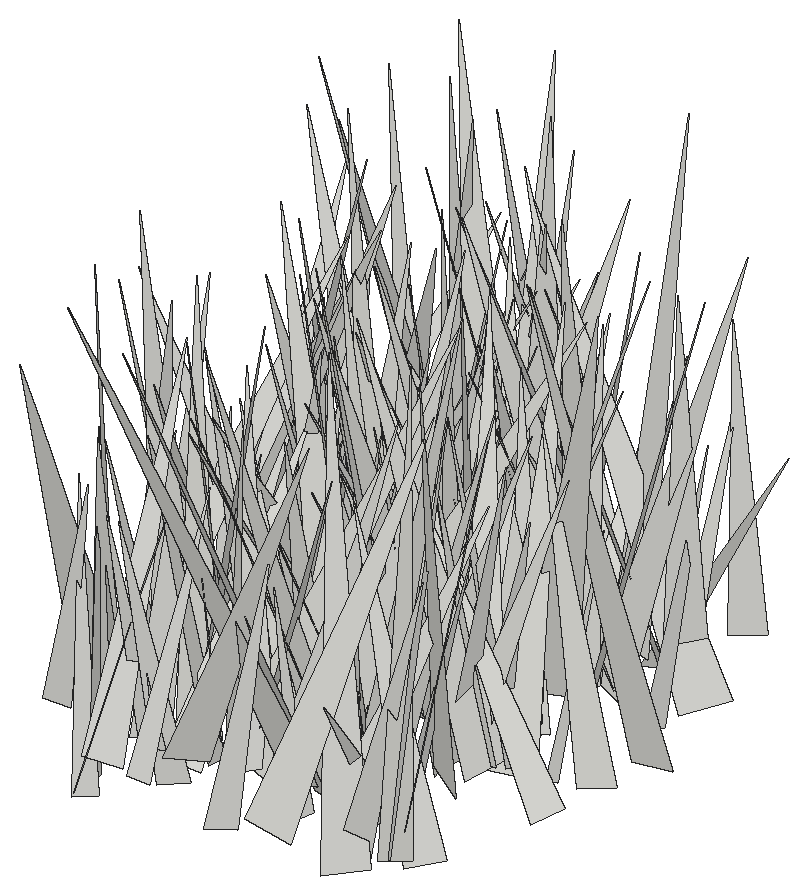
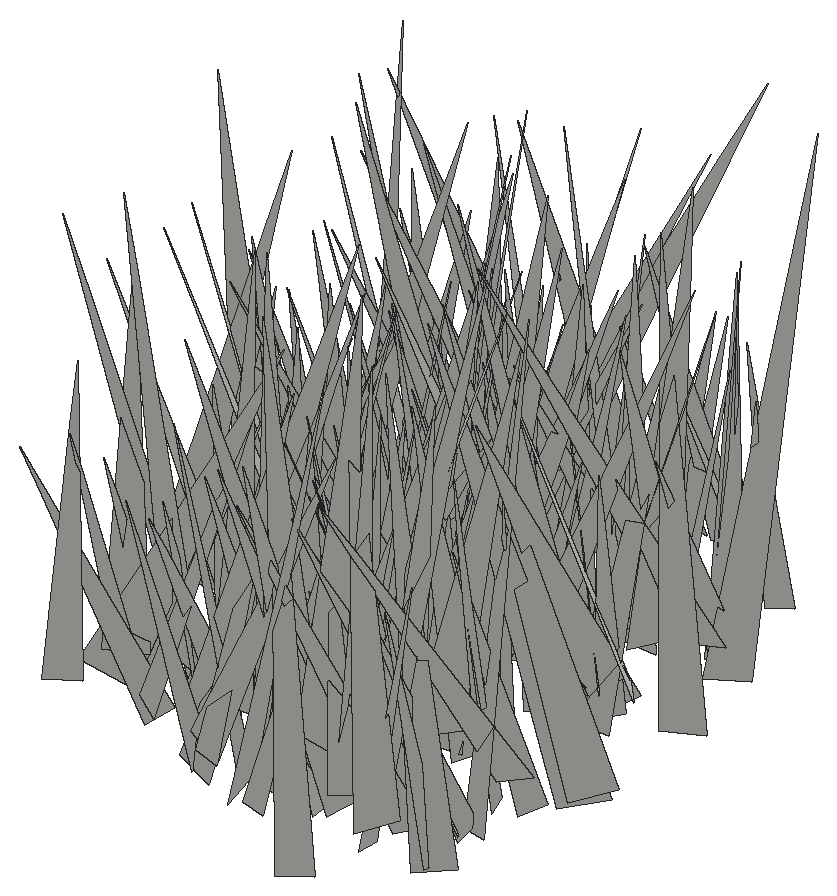
# SketchUp Ruby script. Lengths in inches.
U = 1.inch
M = Sketchup.active_model
def pt(a) = Geom::Point3d.new(a.map { |v| v * U })
def face(e, loops, mat)
  f = e.add_face(loops[0].map { |a| pt(a) })
  loops[1..].each { |l| e.add_face(l.map { |a| pt(a) }).erase! }
  f.material = f.back_material = mat if mat
  f
end
# faces: each face lists its corners as indices into pts; further lists are holes
def faces(e, pts, list, mat = nil) = list.each { |f| face(e, (f[0].is_a?(Array) ? f : [f]).map { |l| l.map { |i| pts[i] } }, mat) }
# xy, xz, yz: faces in a plane at the given z, y or x. An outline is a flat list of corners, or four numbers for a rectangle; further outlines are holes
def ring(l) = l.size == 4 ? [[l[0], l[1]], [l[2], l[1]], [l[2], l[3]], [l[0], l[3]]] : l.each_slice(2).to_a
def flat(e, list, mat, &to3) = list.each { |f| face(e, (f[0].is_a?(Array) ? f : [f]).map { |l| ring(l).map { |u, v| to3.(u, v) } }, mat) }
def xy(e, z, list, mat = nil) = flat(e, list, mat) { |x, y| [x, y, z] }
def xz(e, y, list, mat = nil) = flat(e, list, mat) { |x, z| [x, y, z] }
def yz(e, x, list, mat = nil) = flat(e, list, mat) { |y, z| [x, y, z] }
def lines(e, pts, list) = list.each { |a, b| e.add_line(pt(pts[a]), pt(pts[b])) }
# prism: a flat outline (further loops are holes) pulled along v
def prism(e, loops, v, mat = nil)
  f = face(e, loops, mat); d = Geom::Vector3d.new(v.map { |x| x * U })
  f.pushpull(f.normal.samedirection?(d) ? d.length : -d.length)
end
def box(e, o, s, mat = nil) = prism(e, [[o, [o[0] + s[0], o[1], o[2]], [o[0] + s[0], o[1] + s[1], o[2]], [o[0], o[1] + s[1], o[2]]]], [0, 0, s[2]], mat)
def at(x, y, z, deg = 0) = Geom::Transformation.translation(pt([x, y, z])) * Geom::Transformation.rotation(ORIGIN, Z_AXIS, deg.degrees)
def axes(o, x, y, z) = Geom::Transformation.new([*x, 0, *y, 0, *z, 0, *pt(o).to_a, 1])
def part(name) = M.definitions.add(name)
# library, detail: a bought-in or finely detailed component or shape, given as its bounding box
def library(name, o, s) = part(name).tap { |d| box(d.entities, o, s) }
def detail(e, o, s) = box(e.add_group.entities, o, s)
def put(e, d, t, mat = nil) = e.add_instance(d, t).tap { |i| i.material = mat if mat }
def group(e, t, mat = nil) = e.add_group.tap { |g| g.transformation = t; g.material = mat if mat }.entities
root = M.entities
c1 = part("fur_instance\#9")
p = [[0.8125,0,1.79],[0.67,-0.02,1.48],[0,-0.11,0],[0,0.11,0]]
faces(c1.entities,p,[[0,1,2,3]])
put(root,c1,axes([100.01,75.59,-28.22],[-2.89622,3.26829,0.45856],[3.08153,2.89643,-1.18106],[1.18158,0.4572,4.20415]))
put(root,c1,axes([98.46,79.53,-28.22],[1.17018,-6.95871,1.51726],[-7.0392,-0.89595,1.31981],[1.08411,1.69372,6.93189]))
put(root,c1,axes([100.8125,79.71,-28.22],[-6.13074,4.86156,0.06985],[4.48302,5.69573,-2.94734],[1.88206,2.26926,7.24803]))
put(root,c1,axes([98.97,85.51,-28.22],[3.48145,-1.92251,0.90917],[-2.10367,-3.36896,0.93158],[-0.31179,1.26381,3.86636]))
put(root,c1,axes([99.36,76.44,-28.22],[7.10031,-2.91459,1.55919],[-2.29482,-7.00551,-2.64516],[-2.37902,-1.94118,7.20502]))
put(root,c1,axes([96.93,85.39,-27.1],[2.93254,-6.52755,1.0505],[-6.19008,-2.30697,2.94501],[2.32281,2.09313,6.52193]))
put(root,c1,axes([101.95,73.62,-27.1],[-6.04222,-2.58238,2.07365],[-3.21518,5.60869,-2.38377],[0.79453,3.05796,6.1233]))
put(root,c1,axes([99.51,73.96,-27.1],[1.31397,-3.56018,1.31098],[-3.78942,-1.16427,0.63629],[0.18405,1.44556,3.7412]))
put(root,c1,axes([99.41,87.54,-28.22],[-3.32814,-6.39102,1.50803],[-6.07577,3.63841,2.01068],[2.49085,0.3356,6.91945]))
put(root,c1,axes([100.65,77.48,-28.22],[-4.40075,-1.21691,1.44212],[-0.98766,4.60363,0.87078],[1.60783,-0.50284,4.4821]))
put(root,c1,axes([98.09,84.33,-28.22],[3.6811,-6.05089,2.6185],[-6.53456,-2.94932,2.37094],[0.87715,3.42178,6.67401]))
put(root,c1,axes([99.13,89.62,-28.22],[3.61055,-0.61097,0.20103],[-0.59508,-3.6081,-0.27795],[-0.24409,-0.24103,3.65131]))
put(root,c1,axes([100.23,85.98,-27.1],[-1.46329,-3.87448,2.4887],[-4.52721,1.6881,-0.03379],[0.84239,2.34204,4.14146]))
put(root,c1,axes([101,77.68,-27.1],[-6.55699,2.55506,2.62376],[2.8465,6.94107,0.35432],[2.30431,-1.30376,7.02829]))
put(root,c1,axes([99.91,85.91,-28.22],[3.88099,1.49769,1.22771],[1.56049,-4.04689,0.00388],[-1.14683,-0.43823,4.15995]))
put(root,c1,axes([100.62,80.06,-28.22],[-3.06481,2.41196,1.362],[2.48233,3.29293,-0.24563],[1.22908,-0.63618,3.89234]))
put(root,c1,axes([102.49,85.38,-27.1],[-6.29408,3.56033,1.19684],[3.6784,6.31519,0.55815],[0.76008,-1.07993,7.20971]))
put(root,c1,axes([101.6,75.62,-28.22],[-6.30964,2.41528,1.06239],[1.96226,6.1361,-2.29599],[1.76402,1.81341,6.35402]))
put(root,c1,axes([99.59,87.58,-28.22],[4.13014,0.16234,0.60229],[0.00137,-4.03539,1.07832],[-0.62379,1.06603,3.99019]))
put(root,c1,axes([99.2,86,-27.1],[-0.72981,5.66267,0.18679],[5.27184,0.7477,-2.06932],[2.0757,0.09199,5.32132]))
put(root,c1,axes([100.07,75.69,-28.22],[1.13187,-5.42392,1.09616],[-5.52646,-1.05128,0.50466],[0.2806,1.17367,5.51773]))
put(root,c1,axes([100.58,80.92,-28.22],[-0.42981,-6.03201,0.26249],[-6.01913,0.44871,0.45551],[0.47339,0.22867,6.03012]))
put(root,c1,axes([101.64,83.25,-28.22],[1.9045,4.44389,1.45881],[4.34306,-2.26488,1.22946],[-1.73613,-0.79091,4.67587]))
put(root,c1,axes([102.3,71.78,-28.22],[-4.5545,1.12209,0.15618],[1.0267,4.36161,-1.39615],[0.47894,1.3207,4.4781]))
put(root,c1,axes([101.24,89.93,-28.22],[-3.854,-0.48704,1.31581],[-0.33639,4.05498,0.51565],[1.36213,-0.37663,3.85028]))
put(root,c1,axes([103.07,80.4375,-27.1],[-6.35837,1.48,1.02188],[1.69793,6.17763,1.61781],[0.593,-1.81932,6.3247]))
put(root,c1,axes([101.9,72.71,-28.22],[-4.76219,-1.42096,1.84075],[-1.91994,4.76946,-1.2853],[1.31199,1.82182,4.80058]))
put(root,c1,axes([103.98,75.7,-28.22],[-6.74391,-2.32387,0.77011],[-2.44649,6.31426,-2.37034],[-0.09,2.49068,6.72772]))
put(root,c1,axes([103.53,85.5,-27.1],[-7.58228,1.17889,0.51367],[1.00041,7.33787,-2.07353],[0.80796,1.97752,7.38791]))
put(root,c1,axes([101.72,89.39,-27.1],[-1.16201,-7.65185,1.0654],[-7.72512,1.16361,-0.06847],[0.09162,1.06366,7.73928]))
put(root,c1,axes([98.97,89.85,-28.22],[1.41766,-6.83451,0.48866],[-6.53171,-1.19719,2.20513],[2.07029,0.90294,6.62252]))
put(root,c1,axes([100.91,81.13,-27.1],[0.42201,3.83383,0.13948],[3.79822,-0.3978,-0.55775],[0.53966,-0.19825,3.81644]))
put(root,c1,axes([100.49,90.47,-27.1],[6.63287,-1.89646,1.66739],[-1.83678,-6.83922,-0.47211],[-1.73291,-0.0097,6.88248]))
put(root,c1,axes([102.21,77.53,-27.1],[-3.53666,-0.44387,1.07965],[-0.6619,3.59984,-0.68824],[0.96154,0.84544,3.49732]))
put(root,c1,axes([100.41,80.79,-27.1],[3.23905,1.92957,1.10614],[2.22288,-2.8741,-1.49551],[-0.07469,-1.85863,3.46094]))
put(root,c1,axes([99.86,76.86,-27.1],[0.36828,7.38641,0.21711],[7.15433,-0.30198,-1.86176],[1.84979,-0.30261,7.15741]))
put(root,c1,axes([104.79,86.1,-27.1],[-7.44301,-3.63877,0.95843],[-3.76282,7.20814,-1.85509],[0.01898,2.08796,8.0745]))
put(root,c1,axes([99.76,80.15,-27.1],[4.90909,4.36789,0.50992],[4.39704,-4.86378,-0.66882],[0.06695,-0.83837,6.53684]))
put(root,c1,axes([102.65,76.53,-28.22],[-0.82841,6.75025,1.93378],[7.00258,0.65031,0.72978],[-0.51887,-2.00072,6.76162]))
put(root,c1,axes([102.76,88.64,-27.1],[-6.8831,0.44539,2.18741],[0.27023,7.20464,-0.61666],[2.21588,0.50489,6.86987]))
put(root,c1,axes([100.75,81.3,-27.1],[7.58691,1.58366,1.76713],[1.48707,-7.78642,0.59349],[-1.84915,0.23586,7.72768]))
put(root,c1,axes([101.79,71.97,-28.22],[3.50829,2.33455,0.59392],[2.17247,-3.51961,1.00185],[-1.04078,0.52272,4.09323]))
put(root,c1,axes([102.16,84.0625,-28.22],[-4.55508,3.55475,2.05706],[3.40532,4.98624,-1.07596],[2.29598,-0.34303,5.67691]))
put(root,c1,axes([102.68,72.08,-27.1],[-0.48607,6.36101,0.33267],[6.36907,0.48063,0.1158],[-0.09028,-0.34048,6.37851]))
put(root,c1,axes([101.26,87.1,-27.1],[4.64309,0.99306,0.50279],[0.80416,-4.48393,1.43003],[-0.7696,1.30595,4.52764]))
put(root,c1,axes([103.92,79.26,-27.1],[-2.71204,2.5664,0.21286],[2.56651,2.66825,0.52947],[-0.21147,-0.53003,3.69611]))
put(root,c1,axes([103.74,88.78,-27.1],[-6.05615,5.17907,2.30301],[5.46239,6.23254,0.34836],[1.51293,-1.77094,7.96105]))
put(root,c1,axes([99.84,87.7,-28.22],[4.83025,3.81866,0.07193],[3.65702,-4.5907,-1.86288],[1.10161,-1.50398,5.86882]))
put(root,c1,axes([103.26,77.46,-28.22],[-4.35453,-4.53446,2.05004],[-4.74623,4.60317,0.10013],[1.49574,1.4055,6.28595]))
put(root,c1,axes([102.32,89.62,-27.1],[2.05705,-3.40779,1.21765],[-3.60141,-2.06493,0.30505],[-0.3543,1.20424,3.9688]))
put(root,c1,axes([103.33,73.59,-27.1],[-0.82021,3.34867,1.94688],[3.86928,0.61559,0.57127],[-0.18046,-2.02092,3.4]))
put(root,c1,axes([102.1,88.45,-28.22],[5.08436,-3.96797,0.13679],[-3.71243,-4.83007,-2.12193],[-1.40762,-1.5937,6.0904]))
put(root,c1,axes([103.39,85.71,-27.1],[1.75124,-3.26229,0.83742],[-3.12175,-1.92651,-0.97669],[-1.26432,0.23809,3.57148]))
put(root,c1,axes([103.32,83.34,-28.22],[2.47706,-6.70826,1.39737],[-6.69174,-2.68793,-1.04158],[-1.47445,0.92925,7.07472]))
put(root,c1,axes([104.625,77.02,-27.1],[-5.51822,-0.21879,0.79161],[-0.32668,5.51842,-0.75206],[0.75352,0.79022,5.4711]))
put(root,c1,axes([100.91,88.46,-28.22],[-0.29614,5.30233,1.4786],[4.87042,0.94241,-2.40408],[2.56516,-1.17721,4.73528]))
put(root,c1,axes([103.8125,73.95,-28.22],[1.8151,-3.86013,1.55176],[-3.9232,-2.15155,-0.76319],[-1.38458,1.03602,4.19675]))
put(root,c1,axes([103.68,85.56,-27.1],[3.73526,4.02595,0.93613],[3.5763,-3.78049,1.98866],[-2.07237,0.73241,5.11915]))
put(root,c1,axes([105.92,80.9,-27.1],[-8.22184,1.12863,0.67504],[0.91948,7.98903,-2.15825],[0.94024,2.05661,8.01339]))
put(root,c1,axes([102.15,80.875,-28.22],[2.54415,-5.74451,1.38415],[-5.89364,-2.3587,1.04378],[0.42454,1.68081,6.19537]))
put(root,c1,axes([103.74,83.01,-28.22],[3.56835,-1.26097,2.05366],[-1.59686,-3.9854,0.32755],[-1.80488,1.03305,3.77039]))
put(root,c1,axes([103.29,74.93,-28.22],[-1.51981,5.35977,0.02073],[5.22969,1.48762,-1.21441],[1.17387,0.31183,5.43711]))
put(root,c1,axes([104.28,82.6,-28.22],[3.27442,-5.47757,0.11686],[-5.10679,-3.10069,-2.24625],[-1.98447,-1.05885,5.97327]))
put(root,c1,axes([102.65,85.68,-28.22],[2.11868,-4.0714,0.72457],[-4.11944,-2.00647,0.77101],[0.3627,0.99394,4.52445]))
put(root,c1,axes([102.05,77.57,-27.1],[6.71325,2.37054,1.67819],[2.73448,-6.58312,-1.63968],[-0.97898,-2.13225,6.9281]))
put(root,c1,axes([103.42,80.14,-27.1],[3.51253,-2.51047,1.78394],[-2.89575,-3.6135,0.61652],[-1.0486,1.56939,4.2732]))
put(root,c1,axes([103.29,82.34,-28.22],[3.83893,-0.81047,1.08867],[-0.8917,-3.9684,0.19003],[-1.0232,0.41758,3.91895]))
put(root,c1,axes([102.89,84.32,-28.22],[-2.08812,-6.42397,1.05341],[-6.15561,2.30841,1.87538],[2.11792,0.37569,6.48927]))
put(root,c1,axes([104.98,85.69,-28.22],[-3.89447,-3.70378,1.65585],[-4.00703,3.87088,-0.766],[0.63525,1.71028,5.3196]))
put(root,c1,axes([105.3,80.53,-27.1],[-4.90258,-2.23132,0.87524],[-2.28191,4.95484,-0.15015],[0.73329,0.50088,5.38438]))
put(root,c1,axes([104.13,71.9,-27.1],[0.66695,4.37993,0.08385],[4.36286,-0.67176,0.3871],[-0.39533,-0.02429,4.41347]))
put(root,c1,axes([105.98,89.55,-28.22],[-7.25051,-1.24633,1.39987],[-1.43303,7.2913,-0.93068],[1.20805,1.16894,7.29774]))
put(root,c1,axes([101.79,92.47,-28.22],[-0.39765,-7.51588,0.89638],[-7.02687,0.7002,2.75371],[2.81337,0.68655,7.00455]))
put(root,c1,axes([105.72,85.72,-28.22],[-0.12405,-5.8754,2.10648],[-6.00776,-0.4589,-1.63376],[-1.69244,2.05962,5.64504]))
put(root,c1,axes([104.71,82.61,-27.1],[4.53456,1.85789,3.16607],[2.55783,-5.20835,-0.60709],[-2.63311,-1.85992,4.86266]))
put(root,c1,axes([105.125,76.03,-28.22],[-5.08391,3.17186,1.29588],[3.17676,5.23223,-0.34381],[1.28383,-0.38638,5.98237]))
put(root,c1,axes([105.21,88.73,-27.1],[-4.80805,-4.95386,1.3489],[-5.02147,4.92244,0.17909],[1.0701,0.84054,6.90116]))
put(root,c1,axes([106.16,83.78,-27.1],[-6.18556,-0.57175,1.0735],[-0.94708,5.75521,-2.39186],[0.76312,2.5082,5.73298]))
put(root,c1,axes([104.8125,88.38,-27.1],[-1.18605,7.62635,1.82441],[7.84154,1.15487,0.27022],[0.00582,-1.84431,7.7133]))
put(root,c1,axes([104.64,80.06,-28.22],[-0.42877,3.87256,1.55947],[4.17346,0.35848,0.25729],[-0.1042,-1.57711,3.88772]))
put(root,c1,axes([106.07,79.6,-28.22],[-1.56968,-5.60909,0.11931],[-5.50885,1.51747,-1.1357],[-1.06238,0.41882,5.71278]))
put(root,c1,axes([108.16,83,-28.22],[-3.37764,5.82202,0.02709],[5.22944,3.02002,2.9728],[-2.55923,-1.51283,6.03878]))
put(root,c1,axes([106.44,78.65,-28.22],[-3.07753,7.46975,2.03134],[7.70521,2.74591,1.57617],[-0.74375,-2.46119,7.92363]))
put(root,c1,axes([103.33,86.05,-27.1],[0.04539,-4.24616,1.86431],[-4.44886,0.48634,1.21602],[1.30888,1.80033,4.06857]))
put(root,c1,axes([106.48,76.65,-28.22],[-1.73609,5.26171,0.91511],[5.1615,1.40586,1.70864],[-1.37182,-1.3693,5.27069]))
put(root,c1,axes([103.14,88.54,-28.22],[5.10289,-1.83511,1.25864],[-2.13691,-4.91957,1.49087],[-0.62081,1.84972,5.21387]))
put(root,c1,axes([105.05,90.23,-28.22],[-1.39577,-4.42794,0.41329],[-4.44248,1.40819,0.08395],[0.20461,0.36877,4.64196]))
put(root,c1,axes([105.97,86.81,-27.1],[-6.32088,1.55628,0.92222],[1.03646,5.86264,-2.78949],[1.48264,2.53644,5.88169]))
put(root,c1,axes([107.03,89.91,-27.1],[-1.92463,-5.23066,1.71698],[-5.26178,1.21283,-2.20335],[-1.6191,2.27625,5.1195]))
put(root,c1,axes([103.92,86.35,-27.1],[4.05853,2.67005,1.15678],[2.78357,-4.14094,-0.20805],[-0.84796,-0.81387,4.85361]))
put(root,c1,axes([103.51,89.23,-28.22],[3.71055,0.76796,0.33165],[0.80764,-3.68168,-0.51076],[-0.21789,-0.56867,3.7546]))
put(root,c1,axes([104.12,75.62,-27.1],[-2.04339,-2.88899,0.9747],[-2.5158,2.26047,1.42575],[1.7225,-0.12566,3.23866]))
put(root,c1,axes([108.05,74.67,-27.1],[-2.49506,-7.82927,1.12782],[-7.54738,2.00233,-2.79687],[-2.3678,1.86761,7.7266]))
put(root,c1,axes([104.51,86.65,-27.1],[-4.3896,-2.50757,2.34029],[-2.3133,4.97071,0.98703],[2.5325,0.19407,4.95805]))
put(root,c1,axes([104.32,85.17,-27.1],[3.89284,1.77366,0.49192],[1.64576,-3.86945,0.92782],[-0.82421,0.65077,4.17603]))
put(root,c1,axes([103.48,83.6,-27.1],[-0.9776,-5.25666,1.94415],[-5.10339,1.65068,1.89699],[2.31681,1.41798,4.99896]))
put(root,c1,axes([104.55,77.27,-28.22],[4.75143,0.92242,1.33841],[0.70934,-4.89704,0.85681],[-1.46255,0.62163,4.7637]))
put(root,c1,axes([105.01,79.16,-28.22],[2.16413,-4.87719,1.14426],[-4.95965,-2.26151,-0.2591],[-0.70577,0.93721,5.32947]))
put(root,c1,axes([105.88,73.98,-27.1],[2.53366,4.26731,1.78001],[4.34271,-2.89305,0.75426],[-1.5872,-1.10369,4.90515]))
put(root,c1,axes([106.84,85.59,-27.1],[-4.29612,3.71614,0.38084],[3.69784,4.31285,-0.36964],[0.52979,0.03157,5.66831]))
put(root,c1,axes([108.75,74.52,-27.1],[-4.44374,-5.75342,0.61079],[-5.6055,4.0905,-2.25122],[-1.43294,1.84058,6.91236]))
put(root,c1,axes([107.61,78.83,-27.1],[-6.80477,1.06742,0.77743],[0.9228,6.76292,-1.20833],[0.94457,1.0827,6.78117]))
put(root,c1,axes([106,83.56,-27.1],[-4.51609,-3.87484,0.43498],[-3.47065,4.29803,2.25393],[1.77713,-1.453,5.5072]))
put(root,c1,axes([105.39,85.02,-28.22],[3.85077,0.95797,1.10657],[0.6489,-3.90916,1.12606],[-1.31192,0.87829,3.80501]))
put(root,c1,axes([105.19,83.03,-28.22],[-2.78361,3.37072,1.19614],[3.02117,3.0272,-1.49988],[1.91443,0.12385,4.10617]))
put(root,c1,axes([105.45,88.49,-27.1],[1.282,-6.99581,3.06835],[-7.6361,-1.26107,0.31524],[-0.21483,3.07701,7.10532]))
put(root,c1,axes([107.69,76.68,-28.22],[-1.13695,-6.80591,1.9758],[-6.92615,0.64332,-1.76957],[-1.50086,2.18691,6.66945]))
put(root,c1,axes([108.11,88.5,-27.1],[-4.76226,4.46867,0.77555],[4.53262,4.64929,1.04363],[-0.16086,-1.29026,6.44663]))
put(root,c1,axes([107.16,81.37,-28.22],[-1.01525,-4.25558,0.24661],[-4.20456,0.95799,-0.77812],[-0.70176,0.41691,4.30525]))
put(root,c1,axes([105.1,89.07,-28.22],[5.19652,-2.78136,0.42044],[-2.54268,-5.02221,-1.79688],[-1.20313,-1.39929,5.61347]))
put(root,c1,axes([106.66,77.33,-27.1],[-4.09518,-5.32392,0.52178],[-5.17841,4.11019,1.29512],[1.34181,-0.38619,6.5907]))
put(root,c1,axes([106.54,79.34,-28.22],[-2.5051,-3.46967,0.23869],[-3.39401,2.50314,0.76559],[0.75915,-0.25846,4.21047]))
put(root,c1,axes([107.37,82.12,-28.22],[-2.79772,3.91125,0.86225],[4.00509,2.73873,0.57209],[0.02536,-1.03446,4.77471]))
put(root,c1,axes([107.67,89.53,-28.22],[-3.1075,-6.9448,0.74353],[-6.98342,3.07514,-0.46373],[-0.12218,0.86773,7.5942]))
put(root,c1,axes([107.15,81.47,-27.1],[1.49882,-6.76146,1.59023],[-6.75855,-1.79498,-1.262],[-1.60255,1.24632,6.80963]))
put(root,c1,axes([106.59,90.36,-27.1],[-1.84979,-4.95748,0.73449],[-4.97918,1.90688,0.3307],[0.56907,0.57009,5.281]))
put(root,c1,axes([105.08,87.41,-27.1],[0.03903,6.40601,1.64221],[6.43648,0.34027,-1.48032],[1.51842,-1.60705,6.23275]))
put(root,c1,axes([104.47,73.68,-27.1],[5.13759,-3.83835,0.8309],[-3.9202,-4.93031,1.46363],[0.23526,1.66651,6.24384]))
put(root,c1,axes([108.26,78.82,-27.1],[-6.28358,-3.49392,1.76213],[-3.72095,6.36668,-0.64478],[1.21124,1.43309,7.16066]))
put(root,c1,axes([106.52,72.7,-28.22],[3.28542,-2.52777,1.83261],[-2.97263,-3.34603,0.71392],[-0.95477,1.71946,4.08337]))
put(root,c1,axes([108.55,80.76,-28.22],[-4.54566,0.43172,0.55069],[0.54174,4.46219,0.97364],[0.44289,-1.02717,4.4611]))
put(root,c1,axes([104.56,76.22,-28.22],[1.48421,7.77893,1.22221],[7.56365,-1.06243,-2.42301],[2.19017,-1.60247,7.53948]))
put(root,c1,axes([104.35,81.83,-28.22],[1.86343,6.88556,0.79652],[6.51007,-1.45535,-2.64927],[2.37997,-1.41024,6.62304]))
put(root,c1,axes([106.92,88.34,-28.22],[4.98467,2.72403,1.68688],[2.57744,-5.26236,0.88159],[-1.90334,0.00786,5.61161]))
put(root,c1,axes([108.66,77.03,-28.22],[-6.4254,-4.61842,2.37343],[-5.01235,6.50279,-0.91585],[1.35622,2.15235,7.85982]))
put(root,c1,axes([107.91,74.72,-28.22],[-3.46887,0.5768,0.94943],[0.60796,3.5911,0.03958],[0.92978,-0.19616,3.51628]))
put(root,c1,axes([107.67,86.11,-27.1],[-0.4926,4.67354,0.05511],[4.67276,0.49124,0.10792],[-0.10156,-0.0661,4.69819]))
put(root,c1,axes([106.48,79.76,-27.1],[3.38817,-1.89067,0.4047],[-1.85762,-3.4096,-0.37677],[-0.53632,-0.13453,3.86165]))
put(root,c1,axes([104.58,77.375,-27.1],[6.71484,1.18998,0.43364],[1.2609,-6.06064,-2.89345],[0.11927,-2.92333,6.1752]))
put(root,c1,axes([106.89,76.57,-27.1],[5.00084,3.55671,0.83126],[3.26277,-4.98345,1.69387],[-1.6418,0.92989,5.89825]))
put(root,c1,axes([107.46,77.6,-27.1],[1.47589,3.3854,0.35503],[3.34161,-1.51469,0.55196],[-0.64858,-0.1002,3.65165]))
put(root,c1,axes([107.86,88.125,-27.1],[1.52237,-3.55739,1.37163],[-3.65271,-1.78416,-0.57315],[-1.09275,1.00785,3.82677]))
put(root,c1,axes([105.74,79.33,-28.22],[3.98681,-3.04122,0.56389],[-3.08769,-3.85909,1.01744],[0.18196,1.14894,4.91004]))
put(root,c1,axes([109.42,86.68,-28.22],[2.58278,-6.81445,2.81399],[-6.72051,-3.40212,-2.07037],[-3.03151,1.73634,6.98721]))
put(root,c1,axes([107.83,87.72,-27.1],[0.14601,-6.62439,2.10053],[-6.94709,-0.08453,0.21629],[0.18059,2.1039,6.62247]))
put(root,c1,axes([109.15,79.44,-28.22],[-4.91949,-2.25789,1.34677],[-2.33985,5.06309,-0.05864],[1.19873,0.61667,5.41258]))
put(root,c1,axes([108.59,88.36,-27.1],[2.63611,-2.6678,0.56163],[-2.26437,-2.5776,-1.61563],[-1.51829,-0.78771,3.38467]))
put(root,c1,axes([107.42,77.67,-27.1],[0.16612,7.76506,1.97129],[7.95416,0.07536,-0.96713],[0.95574,-1.97685,7.70638]))
put(root,c1,axes([107.44,77.375,-28.22],[2.79472,-2.37927,0.19168],[-2.37504,-2.80125,-0.14262],[-0.23842,0.01542,3.66757]))
put(root,c1,axes([109.67,89.13,-27.1],[-3.13069,-4.74867,0.6646],[-4.79451,3.11096,-0.35688],[0.06511,0.75154,5.67659]))
put(root,c1,axes([107.81,89.06,-28.22],[4.26152,0.65659,1.09682],[0.47447,-4.35714,0.76482],[-1.18701,0.6156,4.24343]))
put(root,c1,axes([109.875,80.41,-28.22],[-2.69969,6.39263,0.77147],[6.43614,2.65406,0.5304],[-0.19237,-0.91623,6.91901]))
put(root,c1,axes([108.72,86.94,-27.1],[-1.96871,3.37657,0.07437],[3.27614,1.93014,-0.90775],[0.82077,0.39482,3.80171]))
put(root,c1,axes([109.93,86.36,-28.22],[-4.1053,-4.23157,0.31859],[-4.21802,4.11764,0.33835],[0.46467,-0.00766,5.88602]))
put(root,c1,axes([107.41,74.55,-27.1],[1.23681,5.98503,1.54047],[6.1022,-0.934,-1.27052],[0.97821,-1.7408,5.97797]))
put(root,c1,axes([110.89,72.95,-28.22],[-7.08431,2.74004,0.68893],[2.60293,7.0529,-1.28499],[1.09872,0.95845,7.48626]))
put(root,c1,axes([109.98,81,-27.1],[-4.30895,1.90574,0.59057],[1.67064,4.21479,-1.41144],[1.09067,1.07302,4.49519]))
put(root,c1,axes([112.94,86.84,-28.22],[-3.57057,6.8988,1.02898],[6.50769,2.8788,3.28081],[-2.51043,-2.34953,7.04122]))
put(root,c1,axes([109.89,82.52,-28.22],[2.13883,-4.28297,3.06723],[-5.00629,-2.68295,-0.2554],[-1.63976,2.60467,4.7805]))
put(root,c1,axes([108.22,79.89,-27.1],[2.30047,4.4169,0.81433],[4.47004,-2.16262,-0.89782],[0.43686,-1.13065,4.89848]))
put(root,c1,axes([111.53,78.61,-27.1],[-7.04891,1.70289,1.4017],[1.92518,7.04086,1.12767],[1.07622,-1.44158,7.16347]))
put(root,c1,axes([108.5,78.11,-28.22],[3.4607,5.10853,1.2476],[5.25066,-3.43918,-0.48234],[-0.29016,-1.30574,6.15149]))
put(root,c1,axes([110.67,84.1,-27.1],[-4.9436,1.78617,0.77223],[1.56135,4.89918,-1.33648],[1.16143,1.01666,5.08364]))
put(root,c1,axes([112.08,79.14,-27.1],[-5.07583,-0.99149,0.0646],[-0.93064,4.62637,-2.11704],[-0.34804,2.08923,4.7186]))
put(root,c1,axes([111.46,87.08,-28.22],[-3.22494,-3.97651,0.65226],[-4.0077,3.07801,-1.05003],[-0.42001,1.16258,5.01102]))
put(root,c1,axes([108.68,76.95,-27.1],[3.30058,6.51639,2.13105],[6.85171,-3.21879,-0.76942],[-0.24255,-2.25268,7.26396]))
put(root,c1,axes([109.82,86.23,-28.22],[-3.37958,0.77927,1.41196],[0.41341,3.58754,-0.99047],[1.55884,0.73803,3.32382]))
put(root,c1,axes([109.86,83.04,-28.22],[3.13012,3.09581,1.75638],[3.35561,-3.34662,-0.08138],[-1.18695,-1.29717,4.40172]))
put(root,c1,axes([109.7,76.33,-28.22],[3.38324,-1.277,0.34003],[-0.90165,-2.91389,-1.97203],[-0.96612,-1.75247,3.03119]))
put(root,c1,axes([110.29,86.66,-27.1],[2.12447,7.8086,2.15105],[8.03257,-2.31646,0.47574],[-1.03873,-1.94278,8.07844]))
put(root,c1,axes([108.83,81.98,-28.22],[5.77926,4.78065,0.80242],[4.74367,-5.8345,0.5954],[-0.99801,-0.04845,7.47663]))
put(root,c1,axes([111.28,78.78,-27.1],[-0.94166,-4.10224,1.61468],[-4.38512,0.70145,-0.77524],[-0.45421,1.73259,4.13692]))
put(root,c1,axes([111.03,80.34,-28.22],[-1.91608,6.79372,1.10059],[6.8739,1.94553,-0.04218],[0.33984,-1.04766,7.05863]))
put(root,c1,axes([108.91,71.88,-27.1],[-0.63507,6.95916,1.46669],[6.78735,1.03289,-1.962],[2.12438,-1.21968,6.70699]))
put(root,c1,axes([109.42,75.1,-27.1],[0.30593,5.01742,0.69432],[4.86404,-0.09691,-1.44288],[1.4134,-0.75252,4.8152]))
put(root,c1,axes([108.09,82.96,-28.22],[5.98331,3.57339,0.75673],[3.63565,-5.68637,-1.89446],[0.35186,-2.00943,6.70672]))
put(root,c1,axes([112.8,72.82,-27.1],[-7.06937,0.92542,0.80535],[0.55425,6.6114,-2.73188],[1.09444,2.62944,6.58553]))
put(root,c1,axes([112.38,74.73,-28.22],[-3.89894,3.87426,1.21258],[4.05705,3.77806,0.97396],[0.14352,-1.54866,5.40953]))
put(root,c1,axes([109.52,81.21,-28.22],[2.67886,-4.09104,0.57639],[-4.11516,-2.58128,0.80469],[0.36641,0.91951,4.82342]))
put(root,c1,axes([110.41,76.67,-27.1],[3.57631,0.31891,0.97988],[0.16002,-3.66803,0.60973],[-1.01797,0.54376,3.53835]))
put(root,c1,axes([113.36,79.09,-28.22],[-4.58774,2.19144,0.09862],[2.15217,4.45217,1.18567],[-0.42461,-1.11142,4.94408]))
put(root,c1,axes([110.57,78.38,-27.1],[4.80103,-0.44543,1.50068],[-0.59366,-4.99749,0.41591],[-1.44845,0.57184,4.80368]))
put(root,c1,axes([112.47,72.72,-27.1],[3.51213,5.3509,1.08193],[4.75447,-3.63032,2.52063],[-2.68285,0.57134,5.88334]))
put(root,c1,axes([110.61,73.57,-28.22],[4.04203,-2.33275,1.48439],[-2.65208,-4.01454,0.91276],[-0.78205,1.55722,4.57675]))
put(root,c1,axes([111.05,77.28,-27.1],[-3.13728,-6.42445,2.27927],[-6.51063,3.56742,1.09378],[2.01998,1.52023,7.06539]))
put(root,c1,axes([112.17,80.78,-28.22],[1.53322,3.39,0.04746],[3.12816,-1.43461,1.41479],[-1.30727,0.54307,3.44111]))
put(root,c1,axes([110.53,78.82,-27.1],[0.61438,4.77457,1.24038],[4.786,-0.27399,-1.3159],[1.1955,-1.35681,4.63059]))
put(root,c1,axes([111.85,87.27,-27.1],[0.3484,4.1984,0.59349],[4.23915,-0.35779,0.04247],[-0.09183,-0.58788,4.21262]))
put(root,c1,axes([110.14,85.86,-28.22],[2.40948,7.1196,1.80641],[7.28749,-2.07931,-1.52526],[0.91887,-2.17835,7.35989]))
put(root,c1,axes([110.09,83.11,-27.1],[4.60789,-6.31495,1.14074],[-6.41656,-4.51508,0.92427],[0.08686,1.46561,7.76253]))
put(root,c1,axes([112.03,87.09,-27.1],[2.29625,-5.32789,2.30917],[-5.72704,-2.48806,-0.04565],[-0.95905,2.10109,5.80148]))
put(root,c1,axes([113.87,83.24,-28.22],[-1.47229,-7.46087,2.3597],[-7.72207,0.99683,-1.66627],[-1.2659,2.59656,7.41996]))
put(root,c1,axes([113.41,81.26,-28.22],[-2.10663,5.00928,1.58804],[5.23429,1.84857,1.1125],[-0.46582,-1.88217,5.31913]))
put(root,c1,axes([111.6875,74.75,-27.1],[-4.45958,-2.36263,3.46386],[-3.3219,5.07642,-0.81428],[2.55838,2.47306,4.98064]))
put(root,c1,axes([112.42,89.4,-27.1],[2.60909,-3.89298,2.22887],[-4.24925,-2.97119,-0.21539],[-1.4377,1.71676,4.68148]))
put(root,c1,axes([111.64,82.97,-27.1],[5.51365,3.20537,1.24598],[2.89904,-5.59864,1.57419],[-1.84998,0.77981,6.18035]))
put(root,c1,axes([110.29,87.78,-28.22],[4.05513,-1.76427,0.28786],[-1.75227,-3.78191,1.50543],[0.35366,1.49134,4.15818]))
put(root,c1,axes([112.5,85.01,-28.22],[-3.9364,0.91485,1.26316],[0.41585,3.92071,-1.54367],[1.50319,1.31107,3.73488]))
